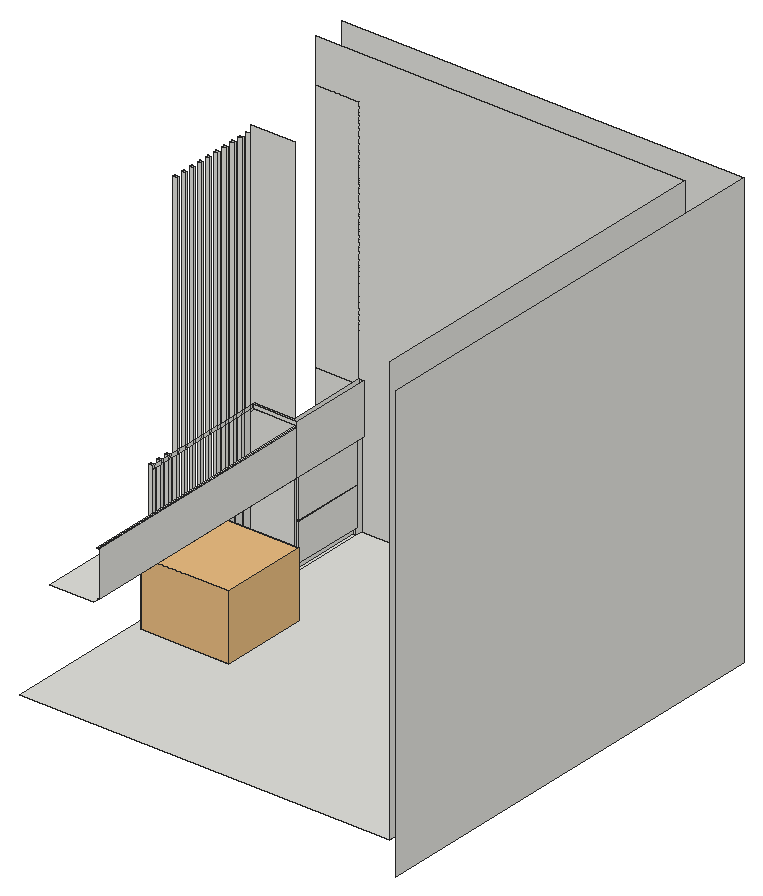
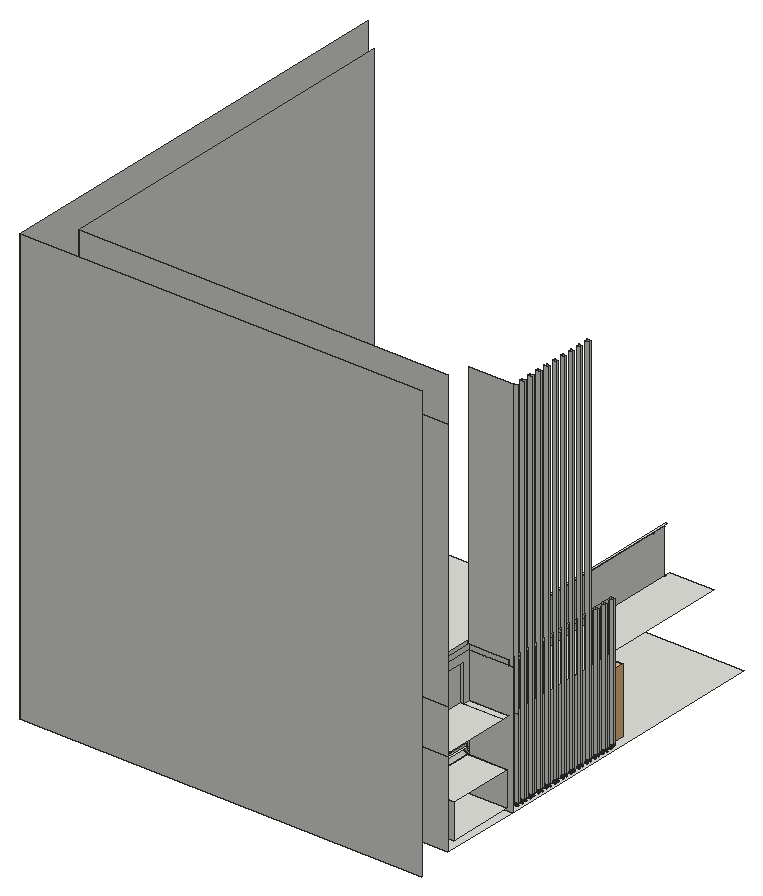
# SketchUp Ruby script. Lengths in inches.
U = 1.inch
M = Sketchup.active_model
def pt(a) = Geom::Point3d.new(a.map { |v| v * U })
def face(e, loops, mat)
  f = e.add_face(loops[0].map { |a| pt(a) })
  loops[1..].each { |l| e.add_face(l.map { |a| pt(a) }).erase! }
  f.material = f.back_material = mat if mat
  f
end
# faces: each face lists its corners as indices into pts; further lists are holes
def faces(e, pts, list, mat = nil) = list.each { |f| face(e, (f[0].is_a?(Array) ? f : [f]).map { |l| l.map { |i| pts[i] } }, mat) }
# xy, xz, yz: faces in a plane at the given z, y or x. An outline is a flat list of corners, or four numbers for a rectangle; further outlines are holes
def ring(l) = l.size == 4 ? [[l[0], l[1]], [l[2], l[1]], [l[2], l[3]], [l[0], l[3]]] : l.each_slice(2).to_a
def flat(e, list, mat, &to3) = list.each { |f| face(e, (f[0].is_a?(Array) ? f : [f]).map { |l| ring(l).map { |u, v| to3.(u, v) } }, mat) }
def xy(e, z, list, mat = nil) = flat(e, list, mat) { |x, y| [x, y, z] }
def xz(e, y, list, mat = nil) = flat(e, list, mat) { |x, z| [x, y, z] }
def yz(e, x, list, mat = nil) = flat(e, list, mat) { |y, z| [x, y, z] }
def lines(e, pts, list) = list.each { |a, b| e.add_line(pt(pts[a]), pt(pts[b])) }
# prism: a flat outline (further loops are holes) pulled along v
def prism(e, loops, v, mat = nil)
  f = face(e, loops, mat); d = Geom::Vector3d.new(v.map { |x| x * U })
  f.pushpull(f.normal.samedirection?(d) ? d.length : -d.length)
end
def box(e, o, s, mat = nil) = prism(e, [[o, [o[0] + s[0], o[1], o[2]], [o[0] + s[0], o[1] + s[1], o[2]], [o[0], o[1] + s[1], o[2]]]], [0, 0, s[2]], mat)
def at(x, y, z, deg = 0) = Geom::Transformation.translation(pt([x, y, z])) * Geom::Transformation.rotation(ORIGIN, Z_AXIS, deg.degrees)
def axes(o, x, y, z) = Geom::Transformation.new([*x, 0, *y, 0, *z, 0, *pt(o).to_a, 1])
def part(name) = M.definitions.add(name)
# library, detail: a bought-in or finely detailed component or shape, given as its bounding box
def library(name, o, s) = part(name).tap { |d| box(d.entities, o, s) }
def detail(e, o, s) = box(e.add_group.entities, o, s)
def put(e, d, t, mat = nil) = e.add_instance(d, t).tap { |i| i.material = mat if mat }
def group(e, t, mat = nil) = e.add_group.tap { |g| g.transformation = t; g.material = mat if mat }.entities
root = M.entities
c1 = library("Round ottoman",[0,0,0],[24.18,24.17,17.98])
xy(root,2,[[9,9,111,9,111,111,21.8,111,21.8,88.73,9,88.73],[9,88.73,21,88.73,21,109,21.8,109,21.8,111,9,111],[21,88.73,21.8,109]])
xy(root,4,[[21,89.04,22,109],[9,90.73,19.875,109],[19.875,90.73,21,109]])
xy(root,13.58,[[9,90.73,19.875,109]])
xy(root,14.23,[[21,89.04,21.8,109],[21.8,89.04,22,109]])
xy(root,14.59,[[21.8,89.04,22,109]])
xy(root,25.62,[[[10,18.02,10,109,21.8,109,21.8,111,22.25,111,22.25,19.91,22.05,19.91,22.05,19.31,22.25,19.31,22.25,18.02],[21,89.04,22,90.73]],[21,89.04,22,90.73],[10,109,21,111]])
xy(root,36,[[21,90.73,22,109]])
xy(root,37.86,[[22.05,19.91,22.25,88.07]])
xy(root,38.47,[[22.05,19.31,22.25,88.07]])
xz(root,53.55,[[9,3.36,10,3.52],[9,3.52,10,39.47]])
xz(root,54.26,[[9,3.29,10,3.36],[9,3.36,10,3.52],[9,3.52,10,39.47]])
xz(root,56.34,[[9,3.36,10,3.52],[9,3.52,10,39.47]])
xz(root,57.04,[[9,3.36,10,3.52],[9,3.52,10,39.47]])
xz(root,59.125,[[9,3.36,10,3.52],[9,3.52,10,39.47]])
xz(root,59.83,[[9,3.36,10,3.52],[9,3.52,10,39.47]])
xz(root,61.91,[[9,3.29,10,3.36],[9,3.36,10,3.52],[9,3.52,10,106.96]])
xz(root,62.62,[[9,3.36,10,3.52],[9,3.52,10,106.96]])
xz(root,64.7,[[9,3.36,10,3.52],[9,3.52,10,106.96]])
xz(root,65.41,[[9,3.29,10,3.36],[9,3.36,10,3.52],[9,3.52,10,106.96]])
xz(root,67.49,[[9,3.36,10,3.52],[9,3.52,10,106.96]])
xz(root,68.19,[[9,3.36,10,3.52],[9,3.52,10,106.96]])
xz(root,70.28,[[9,3.36,10,3.52],[9,3.52,10,106.96]])
xz(root,70.98,[[9,3.36,10,3.52],[9,3.52,10,106.96]])
xz(root,73.0625,[[9,3.36,10,3.52],[9,3.52,10,106.96]])
xz(root,73.77,[[9,3.36,10,3.52],[9,3.52,10,106.96]])
xz(root,75.85,[[9,3.36,10,3.52],[9,3.52,10,106.96]])
xz(root,76.56,[[9,3.36,10,3.52],[9,3.52,10,106.96]])
xz(root,78.64,[[9,3.36,10,3.52],[9,3.52,10,106.96]])
xz(root,79.34,[[9,3.36,10,3.52],[9,3.52,10,106.96]])
xz(root,81.43,[[9,3.36,10,3.52],[9,3.52,10,106.96]])
xz(root,82.13,[[9,3.36,10,3.52],[9,3.52,10,106.96]])
xz(root,84.21,[[9,3.29,10,3.36],[9,3.36,10,3.52],[9,3.52,10,106.96]])
xz(root,84.92,[[9,3.36,10,3.52],[9,3.52,10,106.96]])
xz(root,87,[[9,3.36,10,3.52],[9,3.52,10,25.62],[9,25.62,10,106.96]])
xz(root,88.07,[[22.05,37.86,22.25,38.47],[10,38.47,22.25,39.47]])
xz(root,88.73,[[9,2,21,38],[9,38,10,38,10,39.47,21,39.47,21,108,9,108],[10,38,21,39.47]])
xz(root,89.04,[[21,4,22,14.23],[21,14.23,21.8,14.59],[21,14.59,22,25.62]])
xz(root,90.73,[[9,4,19.875,13.58],[19.875,4,19.875,13.58,21,14.23,21,4],[21,25.62,22,36]])
xz(root,109,[[21,2,21.8,4],[9,4,19.875,13.58],[19.875,4,21.8,4,21.8,14.23,21,14.23,19.875,13.58],[21.8,4,22,14.23],[21.8,14.59,22,25.62],
  [21,25.62,22,36]])
xz(root,111,[[21.8,2,111,2,111,120,9,120,9,108,21,108,21,39.47,22.25,39.47,22.25,25.62,21.8,25.62],[9,2,21.8,2,21.8,25.62,21,25.62,21,25.6,9,25.6],[9,25.6,21,38],[9,25.6,21,38],[21,25.62,21.8,39.47],
  [21.8,25.62,22.25,39.47],[9,38,21,108]])
xz(root,120,[[9,0,120,120]])
yz(root,10,[[55.18,2.4,55.41,2.4,55.47,2.41,55.52,2.42,55.58,2.44,55.63,2.45,55.6875,2.47,55.74,2.5,55.79,2.52,55.89,2.58,55.9375,2.62,55.98,2.65,56.02,2.69,56.0625,2.73,56.1,2.77,56.14,2.82,56.23,2.97,56.27,3.07,56.31,3.18,56.32,3.24,56.33,3.29,56.34,3.36,56.34,25.62,54.26,25.62,54.26,3.29,54.27,3.24,54.29,3.18,54.3,3.125,54.32,3.07,54.34,3.02,54.37,2.97,54.39,2.92,54.42,2.87,54.46,2.82,54.49,2.77,54.61,2.65,54.66,2.62,54.7,2.58,54.8,2.52,54.85,2.5,54.91,2.47,54.96,2.45,55.01,2.44,55.07,2.42],[57.97,2.4,58.2,2.4,58.26,2.41,58.3125,2.42,58.37,2.44,58.42,2.45,58.48,2.47,58.53,2.5,58.58,2.52,58.68,2.58,58.72,2.62,58.77,2.65,58.89,2.77,58.92,2.82,58.96,2.87,58.99,2.92,59.01,2.97,59.04,3.02,59.0625,3.07,59.08,3.125,59.1,3.18,59.11,3.24,59.12,3.29,59.125,3.36,59.125,25.62,57.04,25.62,57.04,3.36,57.05,3.29,57.0625,3.24,57.07,3.18,57.11,3.07,57.15,2.97,57.24,2.82,57.28,2.77,57.4,2.65,57.44,2.62,57.49,2.58,57.59,2.52,57.64,2.5,57.69,2.47,57.75,2.45,57.8,2.44,57.86,2.42,57.91,2.41],[60.76,2.4,60.99,2.4,61.04,2.41,61.1,2.42,61.15,2.44,61.21,2.45,61.26,2.47,61.32,2.5,61.37,2.52,61.47,2.58,61.51,2.62,61.56,2.65,61.68,2.77,61.83,3.02,61.85,3.07,61.87,3.125,61.88,3.18,61.9,3.24,61.91,3.29,61.91,25.62,59.83,25.62,59.83,3.36,59.84,3.29,59.85,3.24,59.86,3.18,59.875,3.125,59.9,3.07,59.94,2.97,60.03,2.82,60.07,2.77,60.15,2.69,60.1875,2.65,60.23,2.62,60.28,2.58,60.33,2.55,60.375,2.52,60.43,2.5,60.48,2.47,60.53,2.45,60.59,2.44,60.64,2.42],[63.54,2.4,63.77,2.4,63.89,2.42,63.94,2.44,64,2.45,64.05,2.47,64.1,2.5,64.15,2.52,64.25,2.58,64.3,2.62,64.34,2.65,64.39,2.69,64.43,2.73,64.46,2.77,64.5,2.82,64.53,2.87,64.5625,2.92,64.59,2.97,64.61,3.02,64.64,3.07,64.65,3.125,64.67,3.18,64.68,3.24,64.69,3.29,64.7,3.36,64.7,25.62,62.62,25.62,62.62,3.36,62.625,3.29,62.64,3.24,62.65,3.18,62.66,3.125,62.68,3.07,62.7,3.02,62.82,2.82,62.86,2.77,62.89,2.73,62.93,2.69,62.98,2.65,63.02,2.62,63.07,2.58,63.11,2.55,63.16,2.52,63.21,2.5,63.27,2.47,63.32,2.45,63.375,2.44,63.43,2.42,63.49,2.41],[66.33,2.4,66.5625,2.4,66.62,2.41,66.67,2.42,66.73,2.44,66.78,2.45,66.84,2.47,66.89,2.5,66.94,2.52,67.04,2.58,67.09,2.62,67.13,2.65,67.25,2.77,67.29,2.82,67.35,2.92,67.4,3.02,67.42,3.07,67.46,3.18,67.47,3.24,67.48,3.29,67.49,3.36,67.49,25.62,65.41,25.62,65.41,3.29,65.42,3.24,65.4375,3.18,65.45,3.125,65.47,3.07,65.49,3.02,65.52,2.97,65.54,2.92,65.57,2.87,65.61,2.82,65.64,2.77,65.76,2.65,65.81,2.62,65.85,2.58,65.95,2.52,66,2.5,66.06,2.47,66.11,2.45,66.16,2.44,66.22,2.42,66.28,2.41],
  [69.12,2.4,69.35,2.4,69.41,2.41,69.46,2.42,69.52,2.44,69.57,2.45,69.625,2.47,69.68,2.5,69.73,2.52,69.83,2.58,69.875,2.62,69.92,2.65,70.04,2.77,70.07,2.82,70.11,2.87,70.14,2.92,70.16,2.97,70.1875,3.02,70.21,3.07,70.25,3.18,70.26,3.24,70.27,3.29,70.28,3.36,70.28,25.62,68.19,25.62,68.19,3.36,68.2,3.29,68.21,3.24,68.22,3.18,68.26,3.07,68.3,2.97,68.39,2.82,68.43,2.77,68.55,2.65,68.59,2.62,68.64,2.58,68.6875,2.55,68.74,2.52,68.79,2.5,68.84,2.47,68.9,2.45,68.95,2.44,69.01,2.42,69.0625,2.41],[71.91,2.4,72.14,2.4,72.19,2.41,72.25,2.42,72.3,2.44,72.36,2.45,72.41,2.47,72.47,2.5,72.52,2.52,72.62,2.58,72.66,2.62,72.71,2.65,72.83,2.77,72.98,3.02,73,3.07,73.02,3.125,73.03,3.18,73.05,3.24,73.06,3.29,73.0625,3.36,73.0625,25.62,70.98,25.62,70.98,3.36,70.99,3.29,71,3.24,71.01,3.18,71.05,3.07,71.09,2.97,71.18,2.82,71.22,2.77,71.34,2.65,71.38,2.62,71.43,2.58,71.53,2.52,71.58,2.5,71.63,2.47,71.68,2.45,71.74,2.44,71.79,2.42],[74.69,2.4,74.92,2.4,75.04,2.42,75.09,2.44,75.15,2.45,75.2,2.47,75.25,2.5,75.3,2.52,75.4,2.58,75.45,2.62,75.49,2.65,75.54,2.69,75.58,2.73,75.61,2.77,75.65,2.82,75.74,2.97,75.76,3.02,75.79,3.07,75.8,3.125,75.82,3.18,75.83,3.24,75.84,3.29,75.85,3.36,75.85,25.62,73.77,25.62,73.77,3.36,73.78,3.29,73.79,3.24,73.8,3.18,73.8125,3.125,73.83,3.07,73.85,3.02,73.91,2.92,73.9375,2.87,73.97,2.82,74.01,2.77,74.04,2.73,74.08,2.69,74.125,2.65,74.17,2.62,74.22,2.58,74.26,2.55,74.3125,2.52,74.36,2.5,74.42,2.47,74.47,2.45,74.53,2.44,74.58,2.42,74.64,2.41],[77.48,2.4,77.71,2.4,77.77,2.41,77.82,2.42,77.88,2.44,77.93,2.45,77.99,2.47,78.04,2.5,78.09,2.52,78.19,2.58,78.24,2.62,78.28,2.65,78.4,2.77,78.4375,2.82,78.47,2.87,78.53,2.97,78.57,3.07,78.61,3.18,78.62,3.24,78.63,3.29,78.64,3.36,78.64,25.62,76.56,25.62,76.56,3.36,76.5625,3.29,76.57,3.24,76.59,3.18,76.6,3.125,76.62,3.07,76.64,3.02,76.67,2.97,76.69,2.92,76.72,2.87,76.76,2.82,76.79,2.77,76.91,2.65,76.96,2.62,77,2.58,77.1,2.52,77.15,2.5,77.21,2.47,77.26,2.45,77.3125,2.44,77.37,2.42,77.43,2.41],[80.27,2.4,80.5,2.4,80.56,2.41,80.61,2.42,80.67,2.44,80.72,2.45,80.78,2.47,80.83,2.5,80.88,2.52,80.98,2.58,81.02,2.62,81.07,2.65,81.15,2.73,81.1875,2.77,81.22,2.82,81.26,2.87,81.29,2.92,81.3125,2.97,81.34,3.02,81.36,3.07,81.4,3.18,81.41,3.24,81.42,3.29,81.43,3.36,81.43,25.62,79.34,25.62,79.34,3.36,79.35,3.29,79.36,3.24,79.375,3.18,79.39,3.125,79.41,3.07,79.45,2.97,79.54,2.82,79.58,2.77,79.7,2.65,79.74,2.62,79.79,2.58,79.89,2.52,79.94,2.5,79.99,2.47,80.05,2.45,80.1,2.44,80.16,2.42,80.21,2.41],
  [83.06,2.4,83.29,2.4,83.34,2.41,83.4,2.42,83.45,2.44,83.51,2.45,83.5625,2.47,83.62,2.5,83.67,2.52,83.77,2.58,83.8125,2.62,83.86,2.65,83.9,2.69,83.9375,2.73,83.98,2.77,84.1,2.97,84.15,3.07,84.17,3.125,84.18,3.18,84.2,3.24,84.21,3.29,84.21,25.62,82.13,25.62,82.13,3.36,82.14,3.29,82.15,3.24,82.16,3.18,82.2,3.07,82.24,2.97,82.33,2.82,82.37,2.77,82.49,2.65,82.53,2.62,82.58,2.58,82.625,2.55,82.68,2.52,82.73,2.5,82.78,2.47,82.83,2.45,82.89,2.44,82.94,2.42],[85.84,2.4,86.07,2.4,86.13,2.41,86.1875,2.42,86.24,2.44,86.3,2.45,86.35,2.47,86.4,2.5,86.45,2.52,86.55,2.58,86.6,2.62,86.64,2.65,86.69,2.69,86.73,2.73,86.76,2.77,86.8,2.82,86.89,2.97,86.91,3.02,86.9375,3.07,86.95,3.125,86.97,3.18,86.98,3.24,86.99,3.29,87,3.36,87,25.62,84.92,25.62,84.92,3.36,84.93,3.29,84.9375,3.24,84.95,3.18,84.96,3.125,84.98,3.07,85,3.02,85.12,2.82,85.16,2.77,85.19,2.73,85.23,2.69,85.28,2.65,85.32,2.62,85.37,2.58,85.41,2.55,85.46,2.52,85.51,2.5,85.57,2.47,85.62,2.45,85.68,2.44,85.73,2.42,85.79,2.41],[53.55,25.62,54.26,38.47],[56.34,25.62,57.04,38.47],[59.125,25.62,59.83,38.47],
  [61.91,25.62,62.62,38.47],[64.7,25.62,65.41,38.47],[67.49,25.62,68.19,38.47],[70.28,25.62,70.98,38.47],[73.0625,25.62,73.77,38.47],
  [75.85,25.62,76.56,38.47],[78.64,25.62,79.34,38.47],[81.43,25.62,82.13,38.47],[84.21,25.62,84.92,38.47],[84.92,25.62,87,38.47],
  [87,38,87,38.47,88.07,38.47,88.07,39.47,88.73,39.47,88.73,38],[53.55,38.47,54.26,39.47],[54.26,38.47,56.34,39.47],[56.34,38.47,57.04,39.47],[57.04,38.47,59.125,39.47],
  [59.125,38.47,59.83,39.47],[59.83,38.47,61.91,39.47],[61.91,38.47,62.62,39.47],[62.62,38.47,64.7,39.47],[64.7,38.47,65.41,39.47],
  [65.41,38.47,67.49,39.47],[67.49,38.47,68.19,39.47],[68.19,38.47,70.28,39.47],[70.28,38.47,70.98,39.47],[70.98,38.47,73.0625,39.47],
  [73.0625,38.47,73.77,39.47],[73.77,38.47,75.85,39.47],[75.85,38.47,76.56,39.47],[76.56,38.47,78.64,39.47],[78.64,38.47,79.34,39.47],
  [79.34,38.47,81.43,39.47],[81.43,38.47,82.13,39.47],[82.13,38.47,84.21,39.47],[84.21,38.47,84.92,39.47],[84.92,38.47,87,39.47],
  [87,38.47,88.07,39.47]])
yz(root,19.875,[[90.73,4,109,13.58]])
yz(root,21,[[88.73,2,109,2,109,4,89.04,4,89.04,25.62,90.73,25.62,90.73,36,109,36,109,25.62,111,25.62,111,38,88.73,38],[89.04,4,90.73,14.23],[88.73,38,111,39.47]])
yz(root,21.8,[[109,2,111,25.62],[89.04,14.23,109,14.59]])
yz(root,22,[[89.04,4,109,14.23],[89.04,14.59,109,14.59,109,36,90.73,36,90.73,25.62,89.04,25.62]])
yz(root,22.25,[[19.91,25.62,88.07,37.86],[88.07,25.62,111,39.47]])
yz(root,111,[[9,2,111,120]])
yz(root,120,[[0,0,120,120]])
p = [[9,54.49,2.77],[9,54.53,2.73],[10,54.53,2.73],[10,54.49,2.77],[9,54.57,2.69],[10,54.57,2.69],
  [9,56.0625,2.73],[9,56.1,2.77],[10,56.1,2.77],[10,56.0625,2.73],[9,57.28,2.77],[9,57.32,2.73],
  [10,57.32,2.73],[10,57.28,2.77],[9,57.36,2.69],[10,57.36,2.69],[9,58.85,2.73],[9,58.89,2.77],
  [10,58.89,2.77],[10,58.85,2.73],[9,60.07,2.77],[9,60.11,2.73],[10,60.11,2.73],[10,60.07,2.77],
  [9,61.64,2.73],[9,61.68,2.77],[10,61.68,2.77],[10,61.64,2.73],[9,62.86,2.77],[9,62.89,2.73],
  [10,62.89,2.73],[10,62.86,2.77],[9,64.43,2.73],[9,64.46,2.77],[10,64.46,2.77],[10,64.43,2.73],
  [9,65.64,2.77],[9,65.68,2.73],[10,65.68,2.73],[10,65.64,2.77],[9,67.21,2.73],[9,67.25,2.77],
  [10,67.25,2.77],[10,67.21,2.73],[9,68.43,2.77],[9,68.47,2.73],[10,68.47,2.73],[10,68.43,2.77],
  [9,70,2.73],[9,70.04,2.77],[10,70.04,2.77],[10,70,2.73],[9,71.22,2.77],[9,71.26,2.73],
  [10,71.26,2.73],[10,71.22,2.77],[9,72.79,2.73],[9,72.83,2.77],[10,72.83,2.77],[10,72.79,2.73],
  [9,74.01,2.77],[9,74.04,2.73],[10,74.04,2.73],[10,74.01,2.77],[9,75.58,2.73],[9,75.61,2.77],
  [10,75.61,2.77],[10,75.58,2.73],[9,76.79,2.77],[9,76.83,2.73],[10,76.83,2.73],[10,76.79,2.77],
  [9,78.36,2.73],[9,78.4,2.77],[10,78.4,2.77],[10,78.36,2.73],[9,79.58,2.77],[9,79.62,2.73],
  [10,79.62,2.73],[10,79.58,2.77],[9,81.15,2.73],[9,81.1875,2.77],[10,81.1875,2.77],[10,81.15,2.73],
  [9,82.37,2.77],[9,82.41,2.73],[10,82.41,2.73],[10,82.37,2.77],[9,83.9375,2.73],[9,83.98,2.77],
  [10,83.98,2.77],[10,83.9375,2.73],[9,85.16,2.77],[9,85.19,2.73],[10,85.19,2.73],[10,85.16,2.77],
  [9,86.73,2.73],[9,86.76,2.77],[10,86.76,2.77],[10,86.73,2.73],[9,54.42,2.87],[9,54.46,2.82],
  [10,54.46,2.82],[10,54.42,2.87],[9,56.14,2.82],[10,56.14,2.82],[9,56.17,2.87],[10,56.17,2.87],
  [9,57.21,2.87],[9,57.24,2.82],[10,57.24,2.82],[10,57.21,2.87],[9,58.92,2.82],[10,58.92,2.82],
  [9,58.96,2.87],[10,58.96,2.87],[9,60,2.87],[9,60.03,2.82],[10,60.03,2.82],[10,60,2.87],
  [9,61.71,2.82],[10,61.71,2.82],[9,61.74,2.87],[10,61.74,2.87],[9,62.79,2.87],[9,62.82,2.82],
  [10,62.82,2.82],[10,62.79,2.87],[9,64.5,2.82],[10,64.5,2.82],[9,64.53,2.87],[10,64.53,2.87],
  [9,65.57,2.87],[9,65.61,2.82],[10,65.61,2.82],[10,65.57,2.87],[9,67.29,2.82],[10,67.29,2.82],
  [9,67.32,2.87],[10,67.32,2.87],[9,68.36,2.87],[9,68.39,2.82],[10,68.39,2.82],[10,68.36,2.87],
  [9,70.07,2.82],[10,70.07,2.82],[9,70.11,2.87],[10,70.11,2.87],[9,71.15,2.87],[9,71.18,2.82],
  [10,71.18,2.82],[10,71.15,2.87],[9,72.86,2.82],[10,72.86,2.82],[9,72.89,2.87],[10,72.89,2.87],
  [9,73.9375,2.87],[9,73.97,2.82],[10,73.97,2.82],[10,73.9375,2.87],[9,75.65,2.82],[10,75.65,2.82],
  [9,75.68,2.87],[10,75.68,2.87],[9,76.72,2.87],[9,76.76,2.82],[10,76.76,2.82],[10,76.72,2.87],
  [9,78.4375,2.82],[10,78.4375,2.82],[9,78.47,2.87],[10,78.47,2.87],[9,79.51,2.87],[9,79.54,2.82],
  [10,79.54,2.82],[10,79.51,2.87],[9,81.22,2.82],[10,81.22,2.82],[9,81.26,2.87],[10,81.26,2.87],
  [9,82.3,2.87],[9,82.33,2.82],[10,82.33,2.82],[10,82.3,2.87],[9,84.01,2.82],[10,84.01,2.82],
  [9,84.04,2.87],[10,84.04,2.87],[9,85.09,2.87],[9,85.12,2.82],[10,85.12,2.82],[10,85.09,2.87],
  [9,86.8,2.82],[10,86.8,2.82],[9,86.83,2.87],[10,86.83,2.87],[9,54.37,2.97],[9,54.39,2.92],
  [10,54.39,2.92],[10,54.37,2.97],[9,56.2,2.92],[10,56.2,2.92],[9,56.23,2.97],[10,56.23,2.97],
  [9,57.15,2.97],[9,57.18,2.92],[10,57.18,2.92],[10,57.15,2.97],[9,58.99,2.92],[10,58.99,2.92],
  [9,59.01,2.97],[10,59.01,2.97],[9,59.94,2.97],[9,59.97,2.92],[10,59.97,2.92],[10,59.94,2.97],
  [9,61.77,2.92],[10,61.77,2.92],[9,61.8,2.97],[10,61.8,2.97],[9,62.73,2.97],[9,62.76,2.92],
  [10,62.76,2.92],[10,62.73,2.97],[9,64.5625,2.92],[10,64.5625,2.92],[9,64.59,2.97],[10,64.59,2.97],
  [9,65.52,2.97],[9,65.54,2.92],[10,65.54,2.92],[10,65.52,2.97],[9,67.35,2.92],[10,67.35,2.92],
  [9,67.375,2.97],[10,67.375,2.97],[9,68.3,2.97],[9,68.33,2.92],[10,68.33,2.92],[10,68.3,2.97],
  [9,70.14,2.92],[10,70.14,2.92],[9,70.16,2.97],[10,70.16,2.97],[9,71.09,2.97],[9,71.12,2.92],
  [10,71.12,2.92],[10,71.09,2.97],[9,72.92,2.92],[10,72.92,2.92],[9,72.95,2.97],[10,72.95,2.97],
  [9,73.88,2.97],[9,73.91,2.92],[10,73.91,2.92],[10,73.88,2.97],[9,75.71,2.92],[10,75.71,2.92],
  [9,75.74,2.97],[10,75.74,2.97],[9,76.67,2.97],[9,76.69,2.92],[10,76.69,2.92],[10,76.67,2.97],
  [9,78.5,2.92],[10,78.5,2.92],[9,78.53,2.97],[10,78.53,2.97],[9,79.45,2.97],[9,79.48,2.92],
  [10,79.48,2.92],[10,79.45,2.97],[9,81.29,2.92],[10,81.29,2.92],[9,81.3125,2.97],[10,81.3125,2.97],
  [9,82.24,2.97],[9,82.27,2.92],[10,82.27,2.92],[10,82.24,2.97],[9,84.07,2.92],[10,84.07,2.92],
  [9,84.1,2.97],[10,84.1,2.97],[9,85.03,2.97],[9,85.06,2.92],[10,85.06,2.92],[10,85.03,2.97],
  [9,86.86,2.92],[10,86.86,2.92],[9,86.89,2.97],[10,86.89,2.97],[9,53.46,3.02],[9,53.49,3.07],
  [10,53.49,3.07],[10,53.46,3.02],[9,54.32,3.07],[9,54.34,3.02],[10,54.34,3.02],[10,54.32,3.07],
  [9,56.25,3.02],[10,56.25,3.02],[9,56.27,3.07],[10,56.27,3.07],[9,57.11,3.07],[9,57.13,3.02],
  [10,57.13,3.02],[10,57.11,3.07],[9,59.04,3.02],[10,59.04,3.02],[9,59.0625,3.07],[10,59.0625,3.07],
  [9,59.9,3.07],[9,59.92,3.02],[10,59.92,3.02],[10,59.9,3.07],[9,61.83,3.02],[10,61.83,3.02],
  [9,61.85,3.07],[10,61.85,3.07],[9,62.68,3.07],[9,62.7,3.02],[10,62.7,3.02],[10,62.68,3.07],
  [9,64.61,3.02],[10,64.61,3.02],[9,64.64,3.07],[10,64.64,3.07],[9,65.47,3.07],[9,65.49,3.02],
  [10,65.49,3.02],[10,65.47,3.07],[9,67.4,3.02],[10,67.4,3.02],[9,67.42,3.07],[10,67.42,3.07],
  [9,68.26,3.07],[9,68.28,3.02],[10,68.28,3.02],[10,68.26,3.07],[9,70.1875,3.02],[10,70.1875,3.02],
  [9,70.21,3.07],[10,70.21,3.07],[9,71.05,3.07],[9,71.07,3.02],[10,71.07,3.02],[10,71.05,3.07],
  [9,72.98,3.02],[10,72.98,3.02],[9,73,3.07],[10,73,3.07],[9,73.83,3.07],[9,73.85,3.02],
  [10,73.85,3.02],[10,73.83,3.07],[9,75.76,3.02],[10,75.76,3.02],[9,75.79,3.07],[10,75.79,3.07],
  [9,76.62,3.07],[9,76.64,3.02],[10,76.64,3.02],[10,76.62,3.07],[9,78.55,3.02],[10,78.55,3.02],
  [9,78.57,3.07],[10,78.57,3.07],[9,79.41,3.07],[9,79.43,3.02],[10,79.43,3.02],[10,79.41,3.07],
  [9,81.34,3.02],[10,81.34,3.02],[9,81.36,3.07],[10,81.36,3.07],[9,82.2,3.07],[9,82.22,3.02],
  [10,82.22,3.02],[10,82.2,3.07],[9,84.125,3.02],[10,84.125,3.02],[9,84.15,3.07],[10,84.15,3.07],
  [9,84.98,3.07],[9,85,3.02],[10,85,3.02],[10,84.98,3.07],[9,86.91,3.02],[10,86.91,3.02],
  [9,86.9375,3.07],[10,86.9375,3.07],[9,53.5,3.125],[10,53.5,3.125],[9,53.52,3.18],[10,53.52,3.18],
  [9,54.29,3.18],[9,54.3,3.125],[10,54.3,3.125],[10,54.29,3.18],[9,56.29,3.125],[10,56.29,3.125],
  [9,56.31,3.18],[10,56.31,3.18],[9,57.07,3.18],[9,57.09,3.125],[10,57.09,3.125],[10,57.07,3.18],
  [9,59.08,3.125],[10,59.08,3.125],[9,59.1,3.18],[10,59.1,3.18],[9,59.86,3.18],[9,59.875,3.125],
  [10,59.875,3.125],[10,59.86,3.18],[9,61.87,3.125],[10,61.87,3.125],[9,61.88,3.18],[10,61.88,3.18],
  [9,62.65,3.18],[9,62.66,3.125],[10,62.66,3.125],[10,62.65,3.18],[9,64.65,3.125],[10,64.65,3.125],
  [9,64.67,3.18],[10,64.67,3.18],[9,65.4375,3.18],[9,65.45,3.125],[10,65.45,3.125],[10,65.4375,3.18],
  [9,67.44,3.125],[10,67.44,3.125],[9,67.46,3.18],[10,67.46,3.18],[9,68.22,3.18],[9,68.24,3.125],
  [10,68.24,3.125],[10,68.22,3.18],[9,70.23,3.125],[10,70.23,3.125],[9,70.25,3.18],[10,70.25,3.18],
  [9,71.01,3.18],[9,71.03,3.125],[10,71.03,3.125],[10,71.01,3.18],[9,73.02,3.125],[10,73.02,3.125],
  [9,73.03,3.18],[10,73.03,3.18],[9,73.8,3.18],[9,73.8125,3.125],[10,73.8125,3.125],[10,73.8,3.18],
  [9,75.8,3.125],[10,75.8,3.125],[9,75.82,3.18],[10,75.82,3.18],[9,76.59,3.18],[9,76.6,3.125],
  [10,76.6,3.125],[10,76.59,3.18],[9,78.59,3.125],[10,78.59,3.125],[9,78.61,3.18],[10,78.61,3.18],
  [9,79.375,3.18],[9,79.39,3.125],[10,79.39,3.125],[10,79.375,3.18],[9,81.38,3.125],[10,81.38,3.125],
  [9,81.4,3.18],[10,81.4,3.18],[9,82.16,3.18],[9,82.18,3.125],[10,82.18,3.125],[10,82.16,3.18],
  [9,84.17,3.125],[10,84.17,3.125],[9,84.18,3.18],[10,84.18,3.18],[9,84.95,3.18],[9,84.96,3.125],
  [10,84.96,3.125],[10,84.95,3.18],[9,86.95,3.125],[10,86.95,3.125],[9,86.97,3.18],[10,86.97,3.18],
  [9,53.53,3.24],[10,53.53,3.24],[9,53.54,3.29],[10,53.54,3.29],[9,54.26,3.29],[9,54.27,3.24],
  [10,54.27,3.24],[10,54.26,3.29],[9,56.32,3.24],[10,56.32,3.24],[9,56.33,3.29],[10,56.33,3.29],
  [9,57.05,3.29],[9,57.0625,3.24],[10,57.0625,3.24],[10,57.05,3.29],[9,59.11,3.24],[10,59.11,3.24],
  [9,59.12,3.29],[10,59.12,3.29],[9,59.84,3.29],[9,59.85,3.24],[10,59.85,3.24],[10,59.84,3.29],
  [9,61.9,3.24],[10,61.9,3.24],[9,61.91,3.29],[10,61.91,3.29],[9,62.625,3.29],[9,62.64,3.24],
  [10,62.64,3.24],[10,62.625,3.29],[9,64.68,3.24],[10,64.68,3.24],[9,64.69,3.29],[10,64.69,3.29],
  [9,65.41,3.29],[9,65.42,3.24],[10,65.42,3.24],[10,65.41,3.29],[9,67.47,3.24],[10,67.47,3.24],
  [9,67.48,3.29],[10,67.48,3.29],[9,68.2,3.29],[9,68.21,3.24],[10,68.21,3.24],[10,68.2,3.29],
  [9,70.26,3.24],[10,70.26,3.24],[9,70.27,3.29],[10,70.27,3.29],[9,70.99,3.29],[9,71,3.24],
  [10,71,3.24],[10,70.99,3.29],[9,73.05,3.24],[10,73.05,3.24],[9,73.06,3.29],[10,73.06,3.29],
  [9,73.78,3.29],[9,73.79,3.24],[10,73.79,3.24],[10,73.78,3.29],[9,75.83,3.24],[10,75.83,3.24],
  [9,75.84,3.29],[10,75.84,3.29],[9,76.5625,3.29],[9,76.57,3.24],[10,76.57,3.24],[10,76.5625,3.29],
  [9,78.62,3.24],[10,78.62,3.24],[9,78.63,3.29],[10,78.63,3.29],[9,79.35,3.29],[9,79.36,3.24],
  [10,79.36,3.24],[10,79.35,3.29],[9,81.41,3.24],[10,81.41,3.24],[9,81.42,3.29],[10,81.42,3.29],
  [9,82.14,3.29],[9,82.15,3.24],[10,82.15,3.24],[10,82.14,3.29],[9,84.2,3.24],[10,84.2,3.24],
  [9,84.21,3.29],[10,84.21,3.29],[9,84.93,3.29],[9,84.9375,3.24],[10,84.9375,3.24],[10,84.93,3.29],
  [9,86.98,3.24],[10,86.98,3.24],[9,86.99,3.29],[10,86.99,3.29],[9,53.55,3.36],[10,53.55,3.36],
  [9,56.34,3.36],[10,56.34,3.36],[9,57.04,3.36],[10,57.04,3.36],[9,59.125,3.36],[10,59.125,3.36],
  [9,59.83,3.36],[10,59.83,3.36],[9,62.62,3.36],[10,62.62,3.36],[9,64.7,3.36],[10,64.7,3.36],
  [9,67.49,3.36],[10,67.49,3.36],[9,68.19,3.36],[10,68.19,3.36],[9,70.28,3.36],[10,70.28,3.36],
  [9,70.98,3.36],[10,70.98,3.36],[9,73.0625,3.36],[10,73.0625,3.36],[9,73.77,3.36],[10,73.77,3.36],
  [9,75.85,3.36],[10,75.85,3.36],[9,76.56,3.36],[10,76.56,3.36],[9,78.64,3.36],[10,78.64,3.36],
  [9,79.34,3.36],[10,79.34,3.36],[9,81.43,3.36],[10,81.43,3.36],[9,82.13,3.36],[10,82.13,3.36],
  [9,84.92,3.36],[10,84.92,3.36],[9,87,3.36],[10,87,3.36],[19.875,90.73,13.58],[21,90.73,14.23],
  [21,109,14.23],[19.875,109,13.58],[10,88.73,25.62],[21,88.73,25.62],[10,90.73,25.62],[21,90.73,25.62]]
faces(root,p,[[0,1,2,3],[1,4,5,2],[6,7,8,9],[10,11,12,13],[11,14,15,12],[16,17,18,19],[20,21,22,23],[24,25,26,27],
  [28,29,30,31],[32,33,34,35],[36,37,38,39],[40,41,42,43],[44,45,46,47],[48,49,50,51],[52,53,54,55],[56,57,58,59],
  [60,61,62,63],[64,65,66,67],[68,69,70,71],[72,73,74,75],[76,77,78,79],[80,81,82,83],[84,85,86,87],[88,89,90,91],
  [92,93,94,95],[96,97,98,99],[100,101,102,103],[101,0,3,102],[7,104,105,8],[104,106,107,105],[108,109,110,111],[109,10,13,110],
  [17,112,113,18],[112,114,115,113],[116,117,118,119],[117,20,23,118],[25,120,121,26],[120,122,123,121],[124,125,126,127],[125,28,31,126],
  [33,128,129,34],[128,130,131,129],[132,133,134,135],[133,36,39,134],[41,136,137,42],[136,138,139,137],[140,141,142,143],[141,44,47,142],
  [49,144,145,50],[144,146,147,145],[148,149,150,151],[149,52,55,150],[57,152,153,58],[152,154,155,153],[156,157,158,159],[157,60,63,158],
  [65,160,161,66],[160,162,163,161],[164,165,166,167],[165,68,71,166],[73,168,169,74],[168,170,171,169],[172,173,174,175],[173,76,79,174],
  [81,176,177,82],[176,178,179,177],[180,181,182,183],[181,84,87,182],[89,184,185,90],[184,186,187,185],[188,189,190,191],[189,92,95,190],
  [97,192,193,98],[192,194,195,193],[196,197,198,199],[197,100,103,198],[106,200,201,107],[200,202,203,201],[204,205,206,207],[205,108,111,206],
  [114,208,209,115],[208,210,211,209],[212,213,214,215],[213,116,119,214],[122,216,217,123],[216,218,219,217],[220,221,222,223],[221,124,127,222],
  [130,224,225,131],[224,226,227,225],[228,229,230,231],[229,132,135,230],[138,232,233,139],[232,234,235,233],[236,237,238,239],[237,140,143,238],
  [146,240,241,147],[240,242,243,241],[244,245,246,247],[245,148,151,246],[154,248,249,155],[248,250,251,249],[252,253,254,255],[253,156,159,254],
  [162,256,257,163],[256,258,259,257],[260,261,262,263],[261,164,167,262],[170,264,265,171],[264,266,267,265],[268,269,270,271],[269,172,175,270],
  [178,272,273,179],[272,274,275,273],[276,277,278,279],[277,180,183,278],[186,280,281,187],[280,282,283,281],[284,285,286,287],[285,188,191,286],
  [194,288,289,195],[288,290,291,289],[292,293,294,295],[296,297,298,299],[297,196,199,298],[202,300,301,203],[300,302,303,301],[304,305,306,307],
  [305,204,207,306],[210,308,309,211],[308,310,311,309],[312,313,314,315],[313,212,215,314],[218,316,317,219],[316,318,319,317],[320,321,322,323],
  [321,220,223,322],[226,324,325,227],[324,326,327,325],[328,329,330,331],[329,228,231,330],[234,332,333,235],[332,334,335,333],[336,337,338,339],
  [337,236,239,338],[242,340,341,243],[340,342,343,341],[344,345,346,347],[345,244,247,346],[250,348,349,251],[348,350,351,349],[352,353,354,355],
  [353,252,255,354],[258,356,357,259],[356,358,359,357],[360,361,362,363],[361,260,263,362],[266,364,365,267],[364,366,367,365],[368,369,370,371],
  [369,268,271,370],[274,372,373,275],[372,374,375,373],[376,377,378,379],[377,276,279,378],[282,380,381,283],[380,382,383,381],[384,385,386,387],
  [385,284,287,386],[290,388,389,291],[388,390,391,389],[293,392,393,294],[392,394,395,393],[396,397,398,399],[397,296,299,398],[302,400,401,303],
  [400,402,403,401],[404,405,406,407],[405,304,307,406],[310,408,409,311],[408,410,411,409],[412,413,414,415],[413,312,315,414],[318,416,417,319],
  [416,418,419,417],[420,421,422,423],[421,320,323,422],[326,424,425,327],[424,426,427,425],[428,429,430,431],[429,328,331,430],[334,432,433,335],
  [432,434,435,433],[436,437,438,439],[437,336,339,438],[342,440,441,343],[440,442,443,441],[444,445,446,447],[445,344,347,446],[350,448,449,351],
  [448,450,451,449],[452,453,454,455],[453,352,355,454],[358,456,457,359],[456,458,459,457],[460,461,462,463],[461,360,363,462],[366,464,465,367],
  [464,466,467,465],[468,469,470,471],[469,368,371,470],[374,472,473,375],[472,474,475,473],[476,477,478,479],[477,376,379,478],[382,480,481,383],
  [480,482,483,481],[484,485,486,487],[485,384,387,486],[390,488,489,391],[488,490,491,489],[394,492,493,395],[492,494,495,493],[496,497,498,499],
  [497,396,399,498],[402,500,501,403],[500,502,503,501],[504,505,506,507],[505,404,407,506],[410,508,509,411],[508,510,511,509],[512,513,514,515],
  [513,412,415,514],[418,516,517,419],[516,518,519,517],[520,521,522,523],[521,420,423,522],[426,524,525,427],[524,526,527,525],[528,529,530,531],
  [529,428,431,530],[434,532,533,435],[532,534,535,533],[536,537,538,539],[537,436,439,538],[442,540,541,443],[540,542,543,541],[544,545,546,547],
  [545,444,447,546],[450,548,549,451],[548,550,551,549],[552,553,554,555],[553,452,455,554],[458,556,557,459],[556,558,559,557],[560,561,562,563],
  [561,460,463,562],[466,564,565,467],[564,566,567,565],[568,569,570,571],[569,468,471,570],[474,572,573,475],[572,574,575,573],[576,577,578,579],
  [577,476,479,578],[482,580,581,483],[580,582,583,581],[584,585,586,587],[585,484,487,586],[490,588,589,491],[588,590,591,589],[494,592,593,495],
  [502,594,595,503],[596,504,507,597],[510,598,599,511],[600,512,515,601],[602,520,523,603],[526,604,605,527],[534,606,607,535],[608,536,539,609],
  [542,610,611,543],[612,544,547,613],[550,614,615,551],[616,552,555,617],[558,618,619,559],[620,560,563,621],[566,622,623,567],[624,568,571,625],
  [574,626,627,575],[628,576,579,629],[630,584,587,631],[590,632,633,591],[634,635,636,637]])
lines(root,p,[[638,639],[640,641]])
put(root,c1,at(11.49,47.78,2))
